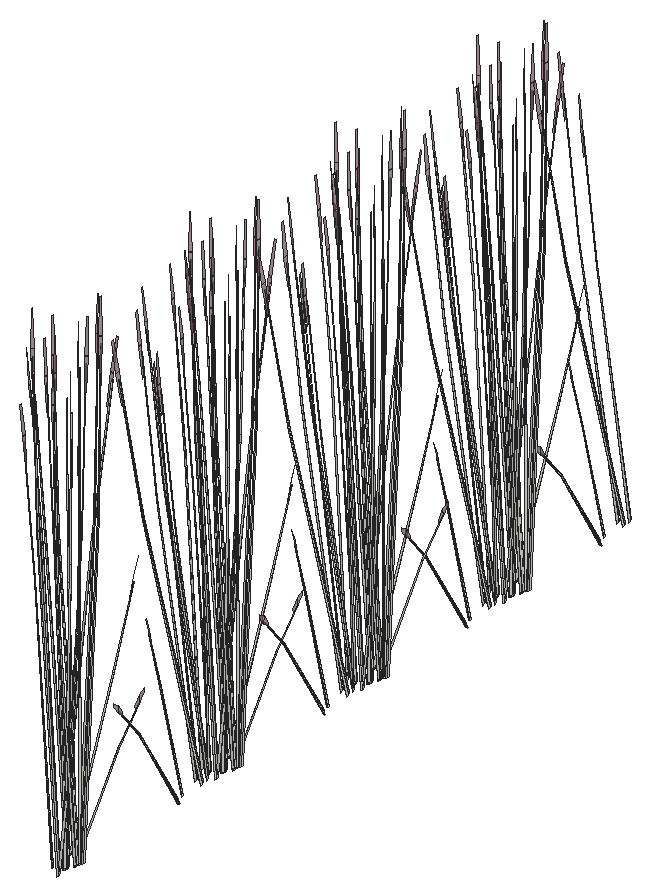
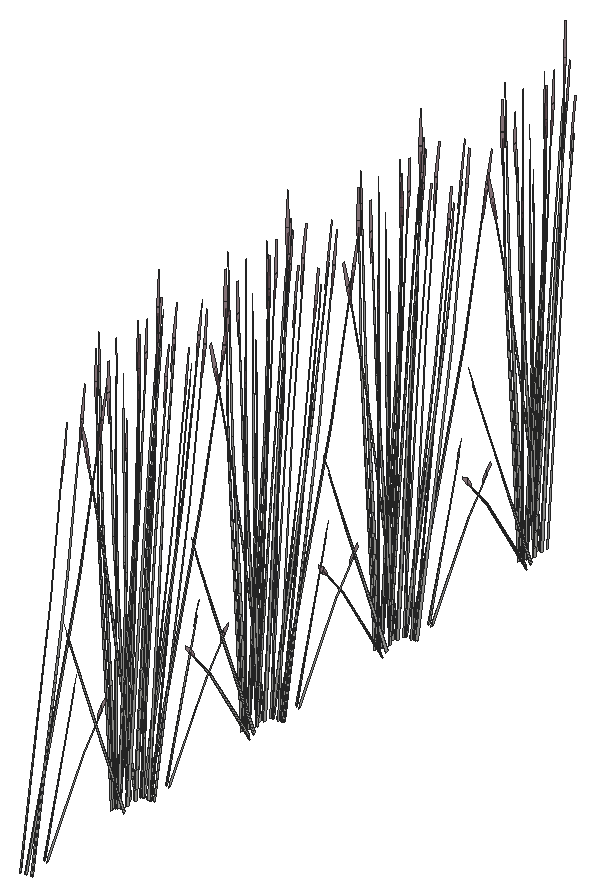
# SketchUp Ruby script. Lengths in inches.
U = 1.inch
M = Sketchup.active_model
def pt(a) = Geom::Point3d.new(a.map { |v| v * U })
def face(e, loops, mat)
  f = e.add_face(loops[0].map { |a| pt(a) })
  loops[1..].each { |l| e.add_face(l.map { |a| pt(a) }).erase! }
  f.material = f.back_material = mat if mat
  f
end
# faces: each face lists its corners as indices into pts; further lists are holes
def faces(e, pts, list, mat = nil) = list.each { |f| face(e, (f[0].is_a?(Array) ? f : [f]).map { |l| l.map { |i| pts[i] } }, mat) }
# xy, xz, yz: faces in a plane at the given z, y or x. An outline is a flat list of corners, or four numbers for a rectangle; further outlines are holes
def ring(l) = l.size == 4 ? [[l[0], l[1]], [l[2], l[1]], [l[2], l[3]], [l[0], l[3]]] : l.each_slice(2).to_a
def flat(e, list, mat, &to3) = list.each { |f| face(e, (f[0].is_a?(Array) ? f : [f]).map { |l| ring(l).map { |u, v| to3.(u, v) } }, mat) }
def xy(e, z, list, mat = nil) = flat(e, list, mat) { |x, y| [x, y, z] }
def xz(e, y, list, mat = nil) = flat(e, list, mat) { |x, z| [x, y, z] }
def yz(e, x, list, mat = nil) = flat(e, list, mat) { |y, z| [x, y, z] }
def lines(e, pts, list) = list.each { |a, b| e.add_line(pt(pts[a]), pt(pts[b])) }
# prism: a flat outline (further loops are holes) pulled along v
def prism(e, loops, v, mat = nil)
  f = face(e, loops, mat); d = Geom::Vector3d.new(v.map { |x| x * U })
  f.pushpull(f.normal.samedirection?(d) ? d.length : -d.length)
end
def box(e, o, s, mat = nil) = prism(e, [[o, [o[0] + s[0], o[1], o[2]], [o[0] + s[0], o[1] + s[1], o[2]], [o[0], o[1] + s[1], o[2]]]], [0, 0, s[2]], mat)
def at(x, y, z, deg = 0) = Geom::Transformation.translation(pt([x, y, z])) * Geom::Transformation.rotation(ORIGIN, Z_AXIS, deg.degrees)
def axes(o, x, y, z) = Geom::Transformation.new([*x, 0, *y, 0, *z, 0, *pt(o).to_a, 1])
def part(name) = M.definitions.add(name)
# library, detail: a bought-in or finely detailed component or shape, given as its bounding box
def library(name, o, s) = part(name).tap { |d| box(d.entities, o, s) }
def detail(e, o, s) = box(e.add_group.entities, o, s)
def put(e, d, t, mat = nil) = e.add_instance(d, t).tap { |i| i.material = mat if mat }
def group(e, t, mat = nil) = e.add_group.tap { |g| g.transformation = t; g.material = mat if mat }.entities
root = M.entities
M.materials.add("LightPink_Translucent").color = [144, 107, 117]
M.materials["LightPink_Translucent"].alpha = 0.75
c1 = part("blade")
p = [[2.15,0.21,22],[0,0.17,0],[0.09,0.45,0],[2.18,0.31,22],[2.29,0.31,22],[0.38,0.45,0],
  [2.48,0.24,33],[2.49,0.24,33],[2.48,0.22,33]]
faces(c1.entities,p,[[0,1,2,3],[4,5,2,3],[6,3,4,7],[8,0,3,6]])
c2 = part("seeds")
p = [[0.3,-0.1,1.38],[-0.01,-0.03,1.59],[-0.01,-0.03,0.03],[0.14,-0.07,-0.07],[0.29,-0.03,3],[0.15,0.01,3.11]]
faces(c2.entities,p,[[0,1,2,3],[1,0,4,5]],"LightPink_Translucent")
c3 = part("blade with seeds")
put(c3.entities,c1,at(0,0,0))
put(c3.entities,c2,axes([2.4,0.25,30.99],[1.5799,-0.05474,1.17369],[-0.12525,1.92788,0.29478],[-0.07173,-0.02425,1.56792]))
put(root,c3,axes([250.64,149.45,0.66],[0,-0.61145,-0.36036],[0.28637,0,0],[0,-0.13926,1.14313]))
put(root,c3,axes([250.64,165.72,0.66],[0,-0.61145,-0.36036],[0.28637,0,0],[0,-0.13926,1.14313]))
put(root,c3,axes([250.64,181.57,0.66],[0,-0.61145,-0.36036],[0.28637,0,0],[0,-0.13926,1.14313]))
put(root,c3,axes([250.64,196.55,0.66],[0,-0.61145,-0.36036],[0.28637,0,0],[0,-0.13926,1.14313]))
put(root,c3,axes([250.76,150.01,0.99],[0,0.61145,0.36036],[-0.28637,0,0],[0,-0.13926,1.14313]))
put(root,c3,axes([250.76,166.28,0.99],[0,0.61145,0.36036],[-0.28637,0,0],[0,-0.13926,1.14313]))
put(root,c3,axes([250.76,182.14,0.99],[0,0.61145,0.36036],[-0.28637,0,0],[0,-0.13926,1.14313]))
put(root,c3,axes([252.07,134.6875,0.78],[-0.15803,-0.61485,-0.03732],[0.26773,-0.34169,0.37456],[-0.06597,0.05854,1.1876]))
put(root,c3,axes([252.07,152.33,0.78],[-0.15803,-0.61485,-0.03732],[0.26773,-0.34169,0.37456],[-0.06597,0.05854,1.1876]))
put(root,c3,axes([252.07,168.6,0.78],[-0.15803,-0.61485,-0.03732],[0.26773,-0.34169,0.37456],[-0.06597,0.05854,1.1876]))
put(root,c3,axes([252.07,184.45,0.78],[-0.15803,-0.61485,-0.03732],[0.26773,-0.34169,0.37456],[-0.06597,0.05854,1.1876]))
put(root,c3,axes([252,134.61,0.66],[-0.23879,-0.15129,-0.22483],[0.06012,-0.53279,0.22483],[-0.04814,0.06144,1.00865]))
put(root,c3,axes([252,152.25,0.66],[-0.23879,-0.15129,-0.22483],[0.06012,-0.53279,0.22483],[-0.04814,0.06144,1.00865]))
put(root,c3,axes([252,168.52,0.66],[-0.23879,-0.15129,-0.22483],[0.06012,-0.53279,0.22483],[-0.04814,0.06144,1.00865]))
put(root,c3,axes([252,184.37,0.66],[-0.23879,-0.15129,-0.22483],[0.06012,-0.53279,0.22483],[-0.04814,0.06144,1.00865]))
put(root,c3,axes([251.38,150.15,1.13],[-0.28825,-0.29175,-0.21117],[0.1388,-0.61578,-0.36291],[-0.00906,-0.15119,1.15913]))
put(root,c3,axes([251.38,166.42,1.13],[-0.28825,-0.29175,-0.21117],[0.1388,-0.61578,-0.36291],[-0.00906,-0.15119,1.15913]))
put(root,c3,axes([251.38,182.28,1.13],[-0.28825,-0.29175,-0.21117],[0.1388,-0.61578,-0.36291],[-0.00906,-0.15119,1.15913]))
put(root,c3,axes([252.13,132.33,1.26],[-0.00699,-0.5757,1.02533],[0.31645,0.14923,0.43413],[-0.07484,0.31502,0.96783]))
put(root,c3,axes([252.13,149.97,1.26],[-0.00699,-0.5757,1.02533],[0.31645,0.14923,0.43413],[-0.07484,0.31502,0.96783]))
put(root,c3,axes([252.13,166.24,1.26],[-0.00699,-0.5757,1.02533],[0.31645,0.14923,0.43413],[-0.07484,0.31502,0.96783]))
put(root,c3,axes([252.13,182.09,1.26],[-0.00699,-0.5757,1.02533],[0.31645,0.14923,0.43413],[-0.07484,0.31502,0.96783]))
put(root,c3,axes([250.86,135.02,1.24],[0.23252,-0.10828,0.04723],[0.05346,0.43623,-0.62638],[-0.01474,0.22082,0.56147]))
put(root,c3,axes([250.86,152.67,1.24],[0.23252,-0.10828,0.04723],[0.05346,0.43623,-0.62638],[-0.01474,0.22082,0.56147]))
put(root,c3,axes([250.86,168.9375,1.24],[0.23252,-0.10828,0.04723],[0.05346,0.43623,-0.62638],[-0.01474,0.22082,0.56147]))
put(root,c3,axes([250.86,184.79,1.24],[0.23252,-0.10828,0.04723],[0.05346,0.43623,-0.62638],[-0.01474,0.22082,0.56147]))
put(root,c3,axes([251.96,133.0625,1.13],[0.02983,0.6977,-0.21117],[-0.31064,0.04219,-0.36291],[-0.0547,0.09294,1.15913]))
put(root,c3,axes([251.96,150.71,1.13],[0.02983,0.6977,-0.21117],[-0.31064,0.04219,-0.36291],[-0.0547,0.09294,1.15913]))
put(root,c3,axes([251.96,166.98,1.13],[0.02983,0.6977,-0.21117],[-0.31064,0.04219,-0.36291],[-0.0547,0.09294,1.15913]))
put(root,c3,axes([251.96,182.83,1.13],[0.02983,0.6977,-0.21117],[-0.31064,0.04219,-0.36291],[-0.0547,0.09294,1.15913]))
put(root,c3,axes([251.25,149.53,0.72],[-0.10512,-0.62701,-0.50685],[0.30279,-0.22582,-0.13303],[-0.01162,-0.21232,1.11879]))
put(root,c3,axes([251.25,165.8,0.72],[-0.10512,-0.62701,-0.50685],[0.30279,-0.22582,-0.13303],[-0.01162,-0.21232,1.11879]))
put(root,c3,axes([251.25,181.66,0.72],[-0.10512,-0.62701,-0.50685],[0.30279,-0.22582,-0.13303],[-0.01162,-0.21232,1.11879]))
put(root,c3,axes([251.25,196.64,0.72],[-0.10512,-0.62701,-0.50685],[0.30279,-0.22582,-0.13303],[-0.01162,-0.21232,1.11879]))
put(root,c3,axes([250.76,149.46,0.66],[0.17867,-0.3815,-0.22483],[0.17867,0.3815,0.22483],[0,-0.12288,1.00865]))
put(root,c3,axes([250.76,165.73,0.66],[0.17867,-0.3815,-0.22483],[0.17867,0.3815,0.22483],[0,-0.12288,1.00865]))
put(root,c3,axes([250.76,181.58,0.66],[0.17867,-0.3815,-0.22483],[0.17867,0.3815,0.22483],[0,-0.12288,1.00865]))
put(root,c3,axes([251.56,146.99,0.74],[-0.17688,0.35078,-0.02825],[-0.16207,-0.38418,-0.1281],[-0.01141,-0.10886,0.42251]))
put(root,c3,axes([251.56,163.26,0.74],[-0.17688,0.35078,-0.02825],[-0.16207,-0.38418,-0.1281],[-0.01141,-0.10886,0.42251]))
put(root,c3,axes([251.56,179.11,0.74],[-0.17688,0.35078,-0.02825],[-0.16207,-0.38418,-0.1281],[-0.01141,-0.10886,0.42251]))
put(root,c3,axes([251.56,194.1,0.74],[-0.17688,0.35078,-0.02825],[-0.16207,-0.38418,-0.1281],[-0.01141,-0.10886,0.42251]))
put(root,c3,axes([251.49,132.81,0.91],[0.32351,0.12883,0.33208],[-0.06584,0.72759,0.13031],[-0.04728,-0.07026,1.15295]))
put(root,c3,axes([251.49,150.45,0.91],[0.32351,0.12883,0.33208],[-0.06584,0.72759,0.13031],[-0.04728,-0.07026,1.15295]))
put(root,c3,axes([251.49,166.72,0.91],[0.32351,0.12883,0.33208],[-0.06584,0.72759,0.13031],[-0.04728,-0.07026,1.15295]))
put(root,c3,axes([251.49,182.57,0.91],[0.32351,0.12883,0.33208],[-0.06584,0.72759,0.13031],[-0.04728,-0.07026,1.15295]))
put(root,c3,axes([251.41,132.68,1.17],[-0.12419,0.55096,0.32471],[-0.25804,-0.26516,-0.15627],[0,-0.12701,1.04254]))
put(root,c3,axes([251.41,150.32,1.17],[-0.12419,0.55096,0.32471],[-0.25804,-0.26516,-0.15627],[0,-0.12701,1.04254]))
put(root,c3,axes([251.41,166.59,1.17],[-0.12419,0.55096,0.32471],[-0.25804,-0.26516,-0.15627],[0,-0.12701,1.04254]))
put(root,c3,axes([251.41,182.44,1.17],[-0.12419,0.55096,0.32471],[-0.25804,-0.26516,-0.15627],[0,-0.12701,1.04254]))
put(root,c3,axes([251.32,133.97,0.99],[0.27504,-0.16229,0.12804],[0.06792,0.60396,0.25465],[-0.02453,-0.088,1.1642]))
put(root,c3,axes([251.32,151.62,0.99],[0.27504,-0.16229,0.12804],[0.06792,0.60396,0.25465],[-0.02453,-0.088,1.1642]))
put(root,c3,axes([251.32,167.88,0.99],[0.27504,-0.16229,0.12804],[0.06792,0.60396,0.25465],[-0.02453,-0.088,1.1642]))
put(root,c3,axes([251.32,183.74,0.99],[0.27504,-0.16229,0.12804],[0.06792,0.60396,0.25465],[-0.02453,-0.088,1.1642]))
put(root,c3,axes([251.67,134.07,0.79],[-0.25804,-0.27452,0],[0.12419,-0.5704,0],[0,0,1.1809]))
put(root,c3,axes([251.67,151.71,0.79],[-0.25804,-0.27452,0],[0.12419,-0.5704,0],[0,0,1.1809]))
put(root,c3,axes([251.67,167.98,0.79],[-0.25804,-0.27452,0],[0.12419,-0.5704,0],[0,0,1.1809]))
put(root,c3,axes([251.67,183.83,0.79],[-0.25804,-0.27452,0],[0.12419,-0.5704,0],[0,0,1.1809]))
put(root,c3,axes([252.27,134.76,0.91],[0.16003,0.61271,0],[-0.26773,0.34169,-0.37456],[-0.06098,0.07782,1.18819]))
put(root,c3,axes([252.27,152.4,0.91],[0.16003,0.61271,0],[-0.26773,0.34169,-0.37456],[-0.06098,0.07782,1.18819]))
put(root,c3,axes([252.27,168.67,0.91],[0.16003,0.61271,0],[-0.26773,0.34169,-0.37456],[-0.06098,0.07782,1.18819]))
put(root,c3,axes([252.27,184.52,0.91],[0.16003,0.61271,0],[-0.26773,0.34169,-0.37456],[-0.06098,0.07782,1.18819]))
put(root,c3,axes([252.14,134.01,0.99],[0.07394,-0.60768,0.12804],[0.27057,0.17197,0.25465],[-0.04674,0.00296,1.1642]))
put(root,c3,axes([252.14,151.65,0.99],[0.07394,-0.60768,0.12804],[0.27057,0.17197,0.25465],[-0.04674,0.00296,1.1642]))
put(root,c3,axes([252.14,167.92,0.99],[0.07394,-0.60768,0.12804],[0.27057,0.17197,0.25465],[-0.04674,0.00296,1.1642]))
put(root,c3,axes([252.14,183.77,0.99],[0.07394,-0.60768,0.12804],[0.27057,0.17197,0.25465],[-0.04674,0.00296,1.1642]))
put(root,c3,axes([252.01,133.2,1.09],[0.1891,0.36737,0.10509],[-0.15773,0.41447,-0.30009],[-0.0439,0.05603,0.91989]))
put(root,c3,axes([252.01,150.84,1.09],[0.1891,0.36737,0.10509],[-0.15773,0.41447,-0.30009],[-0.0439,0.05603,0.91989]))
put(root,c3,axes([252.01,167.11,1.09],[0.1891,0.36737,0.10509],[-0.15773,0.41447,-0.30009],[-0.0439,0.05603,0.91989]))
put(root,c3,axes([252.01,182.96,1.09],[0.1891,0.36737,0.10509],[-0.15773,0.41447,-0.30009],[-0.0439,0.05603,0.91989]))
put(root,c3,axes([251.95,132.75,0.86],[-0.23808,-0.52628,-0.0445],[0.23822,-0.5266,0],[-0.00831,-0.01838,1.27426]))
put(root,c3,axes([251.95,150.39,0.86],[-0.23808,-0.52628,-0.0445],[0.23822,-0.5266,0],[-0.00831,-0.01838,1.27426]))
put(root,c3,axes([251.95,166.66,0.86],[-0.23808,-0.52628,-0.0445],[0.23822,-0.5266,0],[-0.00831,-0.01838,1.27426]))
put(root,c3,axes([251.95,182.51,0.86],[-0.23808,-0.52628,-0.0445],[0.23822,-0.5266,0],[-0.00831,-0.01838,1.27426]))
put(root,c3,axes([252.01,132.93,1.17],[0.27795,-0.03775,0.32471],[0.02514,0.62656,-0.15627],[-0.04976,0.0635,1.04254]))
put(root,c3,axes([252.01,150.57,1.17],[0.27795,-0.03775,0.32471],[0.02514,0.62656,-0.15627],[-0.04976,0.0635,1.04254]))
put(root,c3,axes([252.01,166.84,1.17],[0.27795,-0.03775,0.32471],[0.02514,0.62656,-0.15627],[-0.04976,0.0635,1.04254]))
put(root,c3,axes([252.01,182.69,1.17],[0.27795,-0.03775,0.32471],[0.02514,0.62656,-0.15627],[-0.04976,0.0635,1.04254]))
put(root,c3,axes([252.08,134.37,0.88],[0.32044,0.19874,0.22322],[-0.08017,0.71038,-0.26485],[-0.05304,0.08891,1.19671]))
put(root,c3,axes([252.08,152.01,0.88],[0.32044,0.19874,0.22322],[-0.08017,0.71038,-0.26485],[-0.05304,0.08891,1.19671]))
put(root,c3,axes([252.08,168.28,0.88],[0.32044,0.19874,0.22322],[-0.08017,0.71038,-0.26485],[-0.05304,0.08891,1.19671]))
put(root,c3,axes([252.08,184.13,0.88],[0.32044,0.19874,0.22322],[-0.08017,0.71038,-0.26485],[-0.05304,0.08891,1.19671]))
put(root,c3,axes([251.61,146.5625,0.28],[-0.04293,0.02203,1.27986],[-0.23742,-0.24798,-0.19552],[0.00398,-0.20684,0.218]))
put(root,c3,axes([251.61,162.83,0.28],[-0.04293,0.02203,1.27986],[-0.23742,-0.24798,-0.19552],[0.00398,-0.20684,0.218]))
put(root,c3,axes([251.61,178.68,0.28],[-0.04293,0.02203,1.27986],[-0.23742,-0.24798,-0.19552],[0.00398,-0.20684,0.218]))
put(root,c3,axes([251.61,193.67,0.28],[-0.04293,0.02203,1.27986],[-0.23742,-0.24798,-0.19552],[0.00398,-0.20684,0.218]))
put(root,c3,axes([252.21,134.33,0.99],[0.23955,-0.30573,0.36036],[0.14318,0.54821,0],[-0.05456,0.06963,1.14313]))
put(root,c3,axes([252.21,151.97,0.99],[0.23955,-0.30573,0.36036],[0.14318,0.54821,0],[-0.05456,0.06963,1.14313]))
put(root,c3,axes([252.21,168.24,0.99],[0.23955,-0.30573,0.36036],[0.14318,0.54821,0],[-0.05456,0.06963,1.14313]))
put(root,c3,axes([252.21,184.1,0.99],[0.23955,-0.30573,0.36036],[0.14318,0.54821,0],[-0.05456,0.06963,1.14313]))
put(root,c3,axes([251.47,149.78,0.91],[0.11128,0.68373,0.33208],[-0.31797,0.23776,0.13031],[0.00389,-0.12563,1.15295]))
put(root,c3,axes([251.47,166.05,0.91],[0.11128,0.68373,0.33208],[-0.31797,0.23776,0.13031],[0.00389,-0.12563,1.15295]))
put(root,c3,axes([251.47,181.9,0.91],[0.11128,0.68373,0.33208],[-0.31797,0.23776,0.13031],[0.00389,-0.12563,1.15295]))
put(root,c3,axes([251.41,149.7,0.8],[0.12419,-0.55096,-0.32471],[0.25804,0.26516,0.15627],[0,-0.12701,1.04254]))
put(root,c3,axes([251.41,165.97,0.8],[0.12419,-0.55096,-0.32471],[0.25804,0.26516,0.15627],[0,-0.12701,1.04254]))
put(root,c3,axes([251.41,181.82,0.8],[0.12419,-0.55096,-0.32471],[0.25804,0.26516,0.15627],[0,-0.12701,1.04254]))
put(root,c3,axes([251.41,196.8,0.8],[0.12419,-0.55096,-0.32471],[0.25804,0.26516,0.15627],[0,-0.12701,1.04254]))
put(root,c3,axes([251.73,133.83,0.79],[-0.08351,-0.52716,0],[0.23848,-0.18461,0],[0,0,1.1204]))
put(root,c3,axes([251.73,151.47,0.79],[-0.08351,-0.52716,0],[0.23848,-0.18461,0],[0,0,1.1204]))
put(root,c3,axes([251.73,167.74,0.79],[-0.08351,-0.52716,0],[0.23848,-0.18461,0],[0,0,1.1204]))
put(root,c3,axes([251.73,183.59,0.79],[-0.08351,-0.52716,0],[0.23848,-0.18461,0],[0,0,1.1204]))
put(root,c3,axes([251.43,134.94,0.28],[0.04142,-0.03327,1.27986],[0.24917,0.18313,-0.19552],[0.00729,0.2064,0.218]))
put(root,c3,axes([251.43,152.58,0.28],[0.04142,-0.03327,1.27986],[0.24917,0.18313,-0.19552],[0.00729,0.2064,0.218]))
put(root,c3,axes([251.43,168.85,0.28],[0.04142,-0.03327,1.27986],[0.24917,0.18313,-0.19552],[0.00729,0.2064,0.218]))
